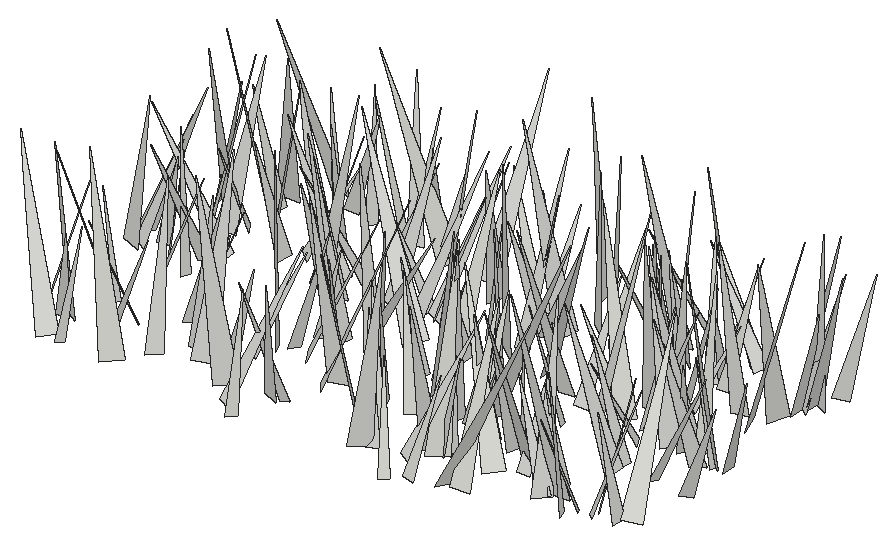
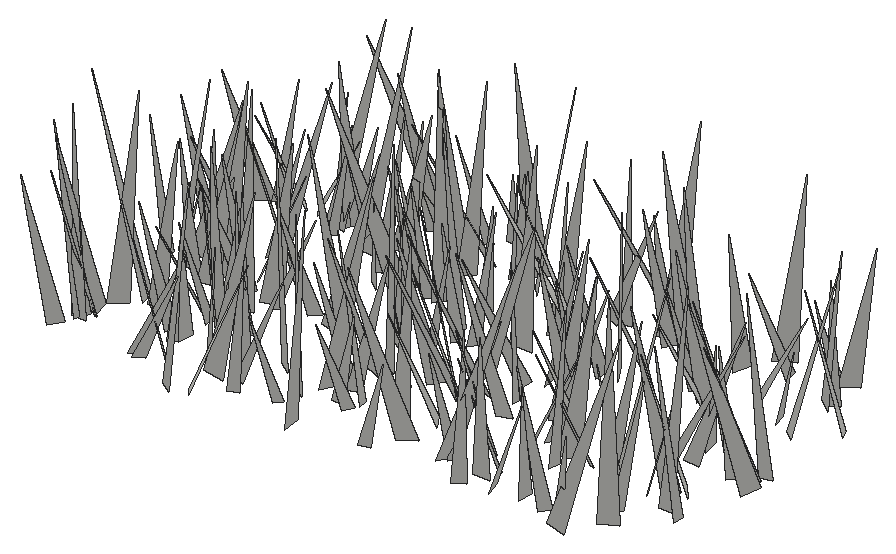
# SketchUp Ruby script. Lengths in inches.
U = 1.inch
M = Sketchup.active_model
def pt(a) = Geom::Point3d.new(a.map { |v| v * U })
def face(e, loops, mat)
  f = e.add_face(loops[0].map { |a| pt(a) })
  loops[1..].each { |l| e.add_face(l.map { |a| pt(a) }).erase! }
  f.material = f.back_material = mat if mat
  f
end
# faces: each face lists its corners as indices into pts; further lists are holes
def faces(e, pts, list, mat = nil) = list.each { |f| face(e, (f[0].is_a?(Array) ? f : [f]).map { |l| l.map { |i| pts[i] } }, mat) }
# xy, xz, yz: faces in a plane at the given z, y or x. An outline is a flat list of corners, or four numbers for a rectangle; further outlines are holes
def ring(l) = l.size == 4 ? [[l[0], l[1]], [l[2], l[1]], [l[2], l[3]], [l[0], l[3]]] : l.each_slice(2).to_a
def flat(e, list, mat, &to3) = list.each { |f| face(e, (f[0].is_a?(Array) ? f : [f]).map { |l| ring(l).map { |u, v| to3.(u, v) } }, mat) }
def xy(e, z, list, mat = nil) = flat(e, list, mat) { |x, y| [x, y, z] }
def xz(e, y, list, mat = nil) = flat(e, list, mat) { |x, z| [x, y, z] }
def yz(e, x, list, mat = nil) = flat(e, list, mat) { |y, z| [x, y, z] }
def lines(e, pts, list) = list.each { |a, b| e.add_line(pt(pts[a]), pt(pts[b])) }
# prism: a flat outline (further loops are holes) pulled along v
def prism(e, loops, v, mat = nil)
  f = face(e, loops, mat); d = Geom::Vector3d.new(v.map { |x| x * U })
  f.pushpull(f.normal.samedirection?(d) ? d.length : -d.length)
end
def box(e, o, s, mat = nil) = prism(e, [[o, [o[0] + s[0], o[1], o[2]], [o[0] + s[0], o[1] + s[1], o[2]], [o[0], o[1] + s[1], o[2]]]], [0, 0, s[2]], mat)
def at(x, y, z, deg = 0) = Geom::Transformation.translation(pt([x, y, z])) * Geom::Transformation.rotation(ORIGIN, Z_AXIS, deg.degrees)
def axes(o, x, y, z) = Geom::Transformation.new([*x, 0, *y, 0, *z, 0, *pt(o).to_a, 1])
def part(name) = M.definitions.add(name)
# library, detail: a bought-in or finely detailed component or shape, given as its bounding box
def library(name, o, s) = part(name).tap { |d| box(d.entities, o, s) }
def detail(e, o, s) = box(e.add_group.entities, o, s)
def put(e, d, t, mat = nil) = e.add_instance(d, t).tap { |i| i.material = mat if mat }
def group(e, t, mat = nil) = e.add_group.tap { |g| g.transformation = t; g.material = mat if mat }.entities
root = M.entities
c1 = part("fur_instance\#9")
p = [[0.8125,0,1.79],[0.67,-0.02,1.48],[0,-0.11,0],[0,0.11,0]]
faces(c1.entities,p,[[0,1,2,3]])
put(root,c1,axes([531.47,279.5,-21.66],[-0.67642,4.08917,0.12939],[3.98053,0.62749,0.97839],[-0.94522,-0.2838,4.0276]))
put(root,c1,axes([507.39,280.67,-21.66],[3.71191,-5.65782,4.04126],[-6.28277,-4.69165,-0.79764],[-2.97818,2.84578,6.7196]))
put(root,c1,axes([518.24,279.79,-21.66],[-3.95695,1.67084,0.9926],[1.45221,4.03835,-1.00857],[1.29152,0.5783,4.17516]))
put(root,c1,axes([532.73,280.46,-21.66],[0.16923,4.07191,1.2027],[4.12697,0.12503,-1.00402],[0.99752,-1.2081,3.94982]))
put(root,c1,axes([527.45,281.94,-21.66],[5.01911,-5.50348,2.14134],[-5.83765,-5.04831,0.7082],[-0.89193,2.07156,7.41473]))
put(root,c1,axes([518.71,283.35,-21.66],[-0.89521,-5.51634,1.09126],[-5.41102,1.14576,1.35291],[1.53027,0.82431,5.42227]))
put(root,c1,axes([501.875,280.69,-21.66],[-4.84886,5.21937,0.60309],[5.25064,4.78392,0.8135],[-0.19034,-0.99462,7.07753]))
put(root,c1,axes([503.04,280.5625,-21.66],[-3.70619,1.07071,1.22273],[0.63141,3.75399,-1.37341],[1.4976,1.06701,3.605]))
put(root,c1,axes([526.24,283.48,-21.66],[-5.36571,-5.00333,1.81378],[-4.95811,5.63559,0.87824],[1.93398,0.5664,7.28374]))
put(root,c1,axes([535.12,281.42,-21.66],[7.55011,-1.58138,0.22082],[-1.59514,-7.42262,1.38345],[0.0711,1.39915,7.58887]))
put(root,c1,axes([515.36,282.86,-21.66],[3.59874,-6.83955,3.08177],[-7.12327,-4.18751,-0.97538],[-2.35281,2.21652,7.66674]))
put(root,c1,axes([501.02,283.32,-21.66],[0.91273,-4.1627,0.50654],[-4.12867,-0.80133,0.85424],[0.734,0.66898,4.1751]))
put(root,c1,axes([516.92,280.75,-21.66],[2.4518,5.85296,0.01413],[5.81055,-2.43218,-0.76857],[0.70347,-0.30989,6.29903]))
put(root,c1,axes([531.23,284.64,-21.66],[5.68928,-3.36377,1.44998],[-3.11585,-5.85243,-1.35122],[-1.92583,-0.46842,6.46971]))
put(root,c1,axes([519.79,283.5625,-21.66],[-0.88602,-4.48963,1.06047],[-4.46813,0.56653,-1.33464],[-1.14769,1.26043,4.37728]))
put(root,c1,axes([505.84,282,-21.66],[4.17653,-0.25853,0.87813],[-0.4857,-4.1025,1.10224],[-0.77592,1.17643,4.03674]))
put(root,c1,axes([536.4,281.39,-21.66],[-1.26821,6.79621,1.34265],[6.86908,1.41065,-0.65215],[0.89826,-1.19212,6.8827]))
put(root,c1,axes([528.29,282.31,-21.66],[-1.05429,4.67357,0.99792],[4.75005,0.91265,0.74413],[-0.52453,-1.12891,4.73287]))
put(root,c1,axes([543.76,283.04,-21.66],[-4.56501,-1.69942,1.47091],[-1.97129,4.62695,-0.77219],[1.07964,1.26263,4.80947]))
put(root,c1,axes([514.65,283.77,-21.66],[3.82808,-2.96393,0.87418],[-3.08142,-3.76593,0.72521],[-0.23226,1.11183,4.78677]))
put(root,c1,axes([538.39,286.5,-21.66],[-2.04467,-7.63412,0.65301],[-7.56547,2.11851,1.07815],[1.21235,0.345,7.82931]))
put(root,c1,axes([542.29,284.84,-21.66],[-1.50167,-7.67594,2.08534],[-7.92089,1.24921,-1.10571],[-0.72669,2.24569,7.7429]))
put(root,c1,axes([501.56,283.66,-21.66],[-3.6941,-4.73944,2.34113],[-5.23892,3.66336,-0.85037],[0.70493,2.38895,5.94858]))
put(root,c1,axes([547.31,284.68,-21.66],[-4.17455,0.44699,1.70239],[0.80041,4.38471,0.81146],[1.56757,-1.04848,4.11925]))
put(root,c1,axes([544.33,284.09,-21.66],[-3.00148,-2.27694,0.1564],[-2.20162,2.82047,-1.1898],[-0.60148,1.03841,3.57459]))
put(root,c1,axes([532.32,284.51,-21.66],[2.08402,3.38406,1.47593],[3.68931,-1.84524,-0.97848],[0.13865,-1.76538,3.85196]))
put(root,c1,axes([541.26,284.22,-21.66],[-2.68831,3.38264,1.06218],[3.54497,2.54168,0.8778],[-0.06058,-1.37662,4.23069]))
put(root,c1,axes([530.9,282.5,-21.66],[2.76171,5.55128,0.00194],[5.48471,-2.72826,-0.95829],[0.85713,-0.42855,6.1258]))
put(root,c1,axes([528.06,283.32,-21.66],[-1.29816,5.29172,0.79515],[5.27739,1.13069,1.0911],[-0.88529,-1.01932,5.33826]))
put(root,c1,axes([508.99,283.17,-21.66],[-5.25856,3.05312,1.43062],[2.8843,5.44607,-1.02073],[1.74617,0.1987,5.99435]))
put(root,c1,axes([510.94,285.32,-21.66],[0.6303,-6.24139,2.24897],[-6.57772,-0.29373,1.02832],[0.86396,2.31708,6.18828]))
put(root,c1,axes([512.25,284.375,-21.66],[-3.47776,6.78239,3.15196],[7.08859,4.09761,-0.99596],[2.38486,-2.28893,7.55669]))
put(root,c1,axes([532.37,284.14,-21.66],[-5.26533,5.42334,2.66225],[5.51698,5.75546,-0.81326],[2.46233,-1.29842,7.51498]))
put(root,c1,axes([505.51,285.72,-21.66],[-2.7303,-2.91554,0.15676],[-2.8364,2.59761,-1.08937],[-0.69267,0.85529,3.84294]))
put(root,c1,axes([541.29,284.04,-21.66],[-5.91196,3.62871,1.99788],[3.48429,6.23911,-1.02156],[2.24027,-0.12769,6.86114]))
put(root,c1,axes([541.53,286.11,-21.66],[-3.71371,1.13934,1.58672],[1.47505,3.87017,0.67337],[1.28063,-1.15373,3.82574]))
put(root,c1,axes([498.09,285.93,-21.66],[4.56554,2.4835,0.72557],[2.58092,-4.47494,-0.92307],[-0.18188,-1.15993,5.11467]))
put(root,c1,axes([545.45,284.02,-21.66],[3.29969,3.36632,0.10349],[3.25213,-3.22241,1.12716],[-0.87548,0.71745,4.57707]))
put(root,c1,axes([532.77,285,-21.66],[1.28068,6.67783,2.12971],[6.86225,-1.63556,1.00185],[-1.42781,-1.87102,6.72532]))
put(root,c1,axes([536.59,284.75,-21.66],[-4.59485,5.55244,0.46156],[5.5505,4.50971,1.00485],[-0.48434,-0.99407,7.1367]))
put(root,c1,axes([535.84,287.96,-21.66],[4.30794,-3.29071,0.86204],[-3.07513,-4.36194,-1.28347],[-1.45447,-0.52435,5.26686]))
put(root,c1,axes([545.42,285,-21.66],[3.89268,2.82638,0.90518],[2.67493,-3.98806,0.94914],[-1.28551,0.26015,4.71599]))
put(root,c1,axes([500.9,288.33,-21.66],[-3.86726,-4.8383,0.71579],[-4.78645,3.93151,0.71436],[1.00566,0.10641,6.1526]))
put(root,c1,axes([534.05,287.73,-21.66],[4.56733,-2.95407,1.62637],[-2.80415,-4.84794,-0.93072],[-1.87305,0.05455,5.35918]))
put(root,c1,axes([525.3,287.41,-21.66],[-4.30625,-1.78107,2.16646],[-1.55574,4.81995,0.87021],[2.33354,-0.07334,4.57807]))
put(root,c1,axes([538.29,285.77,-21.66],[-1.13275,3.97734,1.11963],[3.98013,1.3621,-0.81189],[1.10966,-0.82546,4.05502]))
put(root,c1,axes([521.09,287.69,-21.66],[0.92373,-7.0899,2.33425],[-7.39568,-1.18748,-0.68009],[-1.00963,2.21177,7.11741]))
put(root,c1,axes([530.23,288.39,-21.66],[7.09602,-3.54407,1.49132],[-3.45875,-7.25092,-0.77408],[-1.67974,-0.04148,7.89397]))
put(root,c1,axes([520.56,288.54,-21.66],[-2.364,-4.99525,1.36106],[-4.8414,2.66304,1.36474],[1.83462,0.59091,5.35523]))
put(root,c1,axes([532.5,287.73,-21.66],[4.32257,0.5968,0.21737],[0.63053,-4.21214,-0.97382],[-0.07654,-0.99484,4.25352]))
put(root,c1,axes([508.21,288.06,-21.66],[4.08731,-3.32744,0.79787],[-3.41978,-4.01464,0.77613],[-0.11643,1.10699,5.21302]))
put(root,c1,axes([509.62,287.47,-21.66],[-0.91828,3.53646,1.4047],[3.57282,1.29857,-0.93362],[1.30946,-1.06309,3.53244]))
put(root,c1,axes([531.29,288.7,-21.66],[1.4619,-3.63585,0.57448],[-3.60479,-1.28901,1.01518],[0.74496,0.89757,3.78497]))
put(root,c1,axes([548.03,285.13,-21.66],[-3.4412,6.39637,0.09759],[6.32165,3.41718,-1.06042],[0.97968,0.41743,7.18546]))
put(root,c1,axes([502.64,287.15,-21.66],[-3.94683,-0.00707,0.27926],[-0.08275,3.80753,-1.07302],[0.26682,1.07619,3.79817]))
put(root,c1,axes([514.09,287.3,-21.66],[2.1149,3.97719,0.39309],[3.90996,-1.96694,-1.13523],[0.82754,-0.87089,4.35914]))
put(root,c1,axes([527.41,287.44,-21.66],[-1.32199,4.73147,0.88748],[4.77716,1.17578,0.84759],[-0.59431,-1.0737,4.83901]))
put(root,c1,axes([542.96,289.65,-21.66],[-6.41083,1.14128,1.69671],[1.48537,6.43646,1.28286],[1.40536,-1.59673,6.38401]))
put(root,c1,axes([520.5,286.49,-21.66],[5.97415,4.42308,0.10738],[4.35531,-5.91092,1.16532],[-0.77872,0.87356,7.3414]))
put(root,c1,axes([532.86,288.18,-21.66],[3.50267,-1.34823,2.1537],[-1.97697,-3.75014,0.86764],[-1.59615,1.68627,3.65152]))
put(root,c1,axes([532.64,288.06,-21.66],[-1.16488,5.07104,1.08343],[5.11451,1.30667,-0.61696],[0.85504,-0.90739,5.16641]))
put(root,c1,axes([548.65,290.19,-21.66],[3.25053,-3.28963,0.28157],[-3.26975,-3.15258,0.91484],[0.45796,0.84053,4.53329]))
put(root,c1,axes([517.09,289.33,-21.66],[5.75926,3.61485,0.22209],[3.58079,-5.62103,-1.36658],[0.54262,-1.27375,6.66098]))
put(root,c1,axes([514.87,288.86,-21.66],[-5.7993,-3.05465,2.69516],[-3.68736,5.92923,-1.21419],[1.7315,2.39584,6.44116]))
put(root,c1,axes([508.36,288.34,-21.66],[3.43862,2.40363,0.16823],[2.31203,-3.37399,0.94893],[-0.67841,0.6845,4.08669]))
put(root,c1,axes([515.74,289.65,-21.66],[4.66394,-1.20705,1.00362],[-1.36601,-4.67089,0.73033],[-0.77347,0.97077,4.76192]))
put(root,c1,axes([522.29,290.15,-21.66],[0.36283,-7.33481,3.26148],[-7.98321,-0.67122,-0.62142],[-0.83968,3.21222,7.31744]))
put(root,c1,axes([526.73,291.04,-21.66],[6.91292,1.02767,1.79019],[1.3308,-7.00178,-1.11957],[-1.57792,-1.40299,6.89863]))
put(root,c1,axes([542.87,290.79,-21.66],[-4.85785,0.78834,1.37895],[1.02249,4.94749,0.77364],[1.21552,-1.0112,4.86021]))
put(root,c1,axes([535.15,289.68,-21.66],[1.49909,3.09185,1.25062],[3.12666,-1.78006,0.6529],[-1.16087,-0.8017,3.3735]))
put(root,c1,axes([503.24,290.68,-21.66],[4.3525,2.53578,0.43229],[2.57081,-4.2585,-0.90411],[0.08934,-0.99816,4.9555]))
put(root,c1,axes([531.91,290.41,-21.66],[7.97011,-1.5942,0.50435],[-1.65185,-7.88792,1.1707],[-0.25934,1.24806,8.04323]))
put(root,c1,axes([524.85,291.9,-21.66],[4.20178,-1.75309,2.00996],[-1.5081,-4.65512,-0.90755],[-2.19975,-0.15714,4.46146]))
put(root,c1,axes([545.625,290.49,-21.66],[4.34496,-0.35551,0.43941],[-0.4633,-4.19131,1.19014],[-0.32376,1.22666,4.19388]))
put(root,c1,axes([526.01,292.125,-21.66],[2.52401,-3.24586,0.70539],[-3.32076,-2.44552,0.62916],[0.07602,0.94215,4.0633]))
put(root,c1,axes([516.17,291.78,-21.66],[2.59266,-2.6088,0.97622],[-2.78019,-2.50569,0.68761],[-0.17141,1.18171,3.61316]))
put(root,c1,axes([541.58,293.86,-21.66],[-3.32799,-2.15223,0.18164],[-2.02775,3.22824,1.09879],[0.74386,-0.82886,3.80792]))
put(root,c1,axes([546.8,293.73,-21.66],[0.96308,-5.75121,1.64983],[-5.7805,-1.32563,-1.24675],[-1.54408,1.37555,5.69645]))
put(root,c1,axes([536.19,292.65,-21.66],[-3.92472,-1.58946,0.29836],[-1.61245,3.78584,-1.04222],[-0.12416,1.07696,4.10409]))
put(root,c1,axes([517.86,292.41,-21.66],[-6.43885,-0.2283,0.73687],[-0.34147,6.39798,-1.00159],[0.69173,1.03328,6.36457]))
put(root,c1,axes([498.43,293.88,-21.66],[1.5633,5.69815,3.01797],[6.40687,-1.02237,-1.38843],[0.72737,-3.24142,5.74326]))
put(root,c1,axes([544.76,294.83,-21.66],[3.91329,-2.80057,0.16354],[-2.76188,-3.89534,-0.61821],[-0.49189,-0.40864,4.7723]))
put(root,c1,axes([503.64,295.26,-21.66],[0.77993,-5.26102,0.56712],[-5.12867,-0.89269,-1.22806],[-1.30258,0.36472,5.1748]))
put(root,c1,axes([548.64,294.72,-21.66],[4.67229,-0.63233,0.28263],[-0.57173,-4.60903,-0.86025],[-0.39095,-0.81674,4.63574]))
put(root,c1,axes([503.98,292.79,-21.66],[-5.02502,0.15502,0.9974],[-0.08895,4.97687,-1.22169],[1.00545,1.21508,4.87671]))
put(root,c1,axes([500.14,295.25,-21.66],[2.04033,-4.0488,0.48109],[-4.03745,-1.93127,0.8697],[0.56854,0.81522,4.44965]))
put(root,c1,axes([525.71,295.68,-21.66],[-3.46561,0.71078,2.1355],[1.4755,3.67824,1.17025],[1.69955,-1.74395,3.33859]))
put(root,c1,axes([543.7,294.89,-21.66],[-5.4764,4.5647,2.90915],[5.14181,5.68019,0.76664],[1.69155,-2.48788,7.08799]))
put(root,c1,axes([518.8,294.01,-21.66],[4.72114,-1.50275,0.05764],[-1.46013,-4.53503,1.361],[0.36002,1.31378,4.76394]))
put(root,c1,axes([547.63,294.51,-21.66],[-4.59653,-5.39297,2.39685],[-5.86856,4.49796,-1.13384],[0.62378,2.57709,6.99476]))
put(root,c1,axes([533.8,296.05,-21.66],[-0.89834,-6.55906,1.37521],[-6.65422,0.70817,-0.96916],[-0.7961,1.48213,6.54897]))
put(root,c1,axes([547.69,294.23,-21.66],[-3.7674,-0.4134,0.34529],[-0.49063,3.64055,-0.99453],[0.22227,1.02903,3.6572]))
put(root,c1,axes([501.4,294.21,-21.66],[-2.88957,-1.62735,2.00469],[-2.2228,3.09866,-0.68855],[1.31385,1.66334,3.24403]))
put(root,c1,axes([543.88,296.44,-21.66],[2.81422,-5.9892,1.8303],[-5.99838,-3.15452,-1.09945],[-1.79999,1.14839,6.52546]))
put(root,c1,axes([517.93,296.11,-21.66],[4.34491,0.59069,1.09524],[0.90101,-4.23706,-1.28924],[-0.85828,-1.45776,4.19106]))
put(root,c1,axes([512.7,296.94,-21.66],[2.86729,-4.50295,0.62999],[-4.43501,-2.93396,-0.78577],[-1.00209,0.10064,5.2802]))
put(root,c1,axes([498.9,294.22,-21.66],[2.45412,4.72767,0.6627],[4.74881,-2.3413,-0.8831],[0.48874,-0.99004,5.25297]))
put(root,c1,axes([513.9375,296.49,-21.66],[1.75802,-6.33898,1.96931],[-6.51413,-2.03906,-0.74828],[-1.27556,1.67662,6.53555]))
put(root,c1,axes([529.01,294.93,-21.66],[1.89742,4.59885,2.05217],[4.78177,-2.33318,0.8074],[-1.57969,-1.53878,4.90894]))
put(root,c1,axes([504.62,296.39,-21.66],[-6.1435,0.43905,0.01492],[0.43419,6.03663,1.1429],[-0.06685,-1.14104,6.05221]))
put(root,c1,axes([541.01,295.6,-21.66],[4.40781,-2.35415,1.32075],[-2.57038,-4.43283,0.67704],[-0.82436,1.23418,4.95101]))
put(root,c1,axes([538.34,296.3,-21.66],[-3.99734,1.08155,0.32432],[1.12476,3.91891,0.79421],[0.09918,-0.85212,4.0642]))
put(root,c1,axes([498.08,295.875,-21.66],[6.2285,-2.9564,0.62521],[-3.02175,-6.08711,1.31964],[0.01382,1.46019,6.76705]))
put(root,c1,axes([538.09,293.75,-21.66],[3.95249,6.61953,0.92655],[6.54498,-4.05132,1.02412],[-1.35642,-0.25967,7.64143]))
put(root,c1,axes([539.79,297.64,-21.66],[-0.40221,-7.56998,1.93164],[-7.73436,0.65878,0.97125],[1.10251,1.85984,7.51818]))
put(root,c1,axes([521.65,295.14,-21.66],[-7.18183,4.15456,0.03319],[4.14203,7.15453,0.70461],[-0.3242,-0.62648,8.26695]))
put(root,c1,axes([535.7,295.24,-21.66],[-1.59343,4.55905,1.08338],[4.45907,1.82697,-1.12985],[1.44061,-0.61229,4.69546]))
put(root,c1,axes([530.95,297.67,-21.66],[7.51831,-0.309,0.51299],[-0.23256,-7.46002,-1.08516],[-0.55186,-1.06592,7.446]))
put(root,c1,axes([527.25,297.87,-21.66],[-3.84702,-6.56229,2.86732],[-6.71624,4.43571,1.14075],[2.48541,1.82909,7.52076]))
put(root,c1,axes([538.89,295.8125,-21.66],[2.27452,-5.56414,4.58515],[-6.58849,-3.55674,-1.04785],[-2.92831,3.68058,5.91904]))
put(root,c1,axes([541.07,295.83,-21.66],[4.54007,-1.04122,1.07478],[-1.33062,-4.37982,1.37772],[-0.68465,1.60765,4.44952]))
put(root,c1,axes([545.71,295.54,-21.66],[0.35449,6.1752,1.09899],[6.2119,-0.49795,0.79425],[-0.86782,-1.04187,6.13416]))
put(root,c1,axes([507.69,298.61,-21.66],[-4.50462,1.14541,2.32905],[1.86637,4.67145,1.31236],[1.80364,-1.97324,4.45884]))
put(root,c1,axes([512.69,298.7,-21.66],[-6.22259,1.31552,1.1088],[1.51746,6.15727,1.21077],[0.81078,-1.42761,6.24382]))
put(root,c1,axes([541.85,296.71,-21.66],[-4.80614,1.67739,0.07303],[1.63862,4.73444,-0.90443],[0.36591,0.83033,5.00945]))
put(root,c1,axes([513.59,299.72,-21.66],[-4.70083,-1.74871,0.0814],[-1.70109,4.61801,0.97093],[0.41342,-0.88228,4.92068]))
put(root,c1,axes([512.04,297.14,-21.66],[6.62959,-1.41825,2.66639],[-1.99694,-6.88369,1.30369],[-2.26567,1.91728,6.65307]))
put(root,c1,axes([519.67,299.29,-21.66],[-3.46593,0.7925,0.89611],[1.04093,3.35143,1.06213],[0.58952,-1.25841,3.39303]))
put(root,c1,axes([520.2,296.52,-21.66],[2.81698,6.47491,0.35167],[6.46114,-2.77024,-0.75032],[0.54938,-0.62035,7.02117]))
put(root,c1,axes([523.62,297.37,-21.66],[-3.09006,5.24053,1.65653],[5.13422,3.43055,-1.27548],[1.9614,-0.72379,5.94851]))
put(root,c1,axes([506.57,299.3,-21.66],[-6.42891,-4.93695,1.78859],[-5.18873,6.40682,-0.96596],[0.80598,1.86616,8.04806]))
put(root,c1,axes([503.27,300.42,-21.66],[-3.15969,-2.10838,0.70871],[-1.88389,3.19122,1.09464],[1.18257,-0.54957,3.6374]))
put(root,c1,axes([540.09,299.91,-21.66],[0.10364,-5.95888,1.80759],[-6.13378,0.21397,1.05707],[1.07352,1.79787,5.86529]))
put(root,c1,axes([521.94,297.48,-21.66],[5.36611,5.59511,2.05394],[5.5109,-5.71038,1.15783],[-2.27022,-0.63666,7.66549]))
put(root,c1,axes([520.3,298.75,-21.66],[4.29759,3.17988,0.45483],[3.21134,-4.23507,-0.73441],[0.07624,-0.86047,5.29543]))
put(root,c1,axes([517.2,298.18,-21.66],[0.34617,6.42334,1.62872],[6.51894,-0.03728,-1.2385],[1.18972,-1.66468,6.31231]))
put(root,c1,axes([510.375,299.8,-21.66],[-3.35147,5.54659,2.9979],[6.27053,3.28643,0.92965],[0.65767,-3.06906,6.41348]))
put(root,c1,axes([500.9,301.36,-21.66],[-1.7083,-7.51191,1.45388],[-7.48357,1.95063,1.28533],[1.59333,1.10775,7.59572]))
put(root,c1,axes([510.85,297.48,-21.66],[4.46685,2.95329,0.59597],[2.75098,-4.43263,1.34675],[-1.2285,0.81223,5.18275]))
put(root,c1,axes([539.26,298.79,-21.66],[-4.67336,-1.61213,2.14084],[-2.03116,4.93814,-0.71533],[1.7483,1.42769,4.89159]))
put(root,c1,axes([502.27,299.17,-21.66],[-0.87926,6.56228,2.62812],[6.83144,1.46959,-1.38397],[1.81713,-2.34956,6.47466]))
put(root,c1,axes([525.14,298.42,-21.66],[2.28996,3.33239,0.84649],[3.03653,-2.43723,1.38011],[-1.61271,0.14282,3.80053]))
put(root,c1,axes([546.94,302.08,-21.66],[6.05759,-4.04132,1.47541],[-3.82561,-6.22554,-1.34569],[-1.96821,-0.33746,7.15653]))
put(root,c1,axes([545.92,300.32,-21.66],[7.78659,2.72532,1.24866],[2.87625,-7.77148,-0.97412],[-0.84485,-1.33952,8.19204]))
put(root,c1,axes([508.52,299.76,-21.66],[2.58495,3.56171,0.23056],[3.43761,-2.40789,-1.34382],[0.96012,-0.96809,4.1907]))
put(root,c1,axes([527.24,301.65,-21.66],[2.70621,-3.86796,1.26709],[-3.69816,-2.97221,-1.17466],[-1.70008,0.30833,4.57219]))
put(root,c1,axes([510.52,301.28,-21.66],[5.22033,-0.21574,2.13038],[0.1303,-5.5713,-0.88347],[-2.13731,-0.86658,5.14955]))
put(root,c1,axes([501.4,298.52,-21.66],[4.49985,4.45709,1.03745],[4.28289,-4.6143,1.2473],[-1.61209,0.1822,6.20956]))
put(root,c1,axes([541.65,299.67,-21.66],[1.90499,3.12749,0.05078],[3.06447,-1.8542,-0.76405],[0.62675,-0.43991,3.5814]))
put(root,c1,axes([520.53,298.56,-21.66],[1.99959,6.47326,0.24716],[6.43471,-1.95494,-0.85747],[0.74746,-0.48749,6.72058]))
put(root,c1,axes([544.51,301.06,-21.66],[-0.07394,-6.12578,2.47714],[-6.56947,-0.19789,-0.68546],[-0.70961,2.47033,6.08776]))
put(root,c1,axes([499.51,301.83,-21.66],[5.83398,1.13984,1.03884],[1.35175,-5.73614,-1.2974],[-0.74243,-1.48703,5.80098]))
put(root,c1,axes([527.8,301.2,-21.66],[3.87779,-2.1954,0.31482],[-2.2129,-3.78759,0.8446],[0.14815,0.88911,4.37535]))
put(root,c1,axes([540.71,300.22,-21.66],[4.041,0.55824,1.1889],[0.26805,-4.11576,1.02147],[-1.28579,0.89645,3.94942]))
put(root,c1,axes([532.84,302.01,-21.66],[-4.52397,-6.09316,3.51067],[-6.34353,5.33763,1.08955],[3.03497,2.07386,7.51038]))
put(root,c1,axes([522.19,303.03,-21.66],[5.38586,-3.00561,1.16634],[-2.8404,-5.49795,-1.05176],[-1.52519,-0.37466,6.07741]))
put(root,c1,axes([528.85,302.18,-21.66],[-7.80525,1.8691,2.4402],[2.24771,8.01322,1.05174],[2.09664,-1.63243,7.95672]))
put(root,c1,axes([537.33,300.34,-21.66],[-3.18847,2.06393,0.29466],[1.98964,3.17316,-0.69666],[0.62286,0.42918,3.73374]))
put(root,c1,axes([527.66,298.9,-21.66],[1.84381,6.83005,0.32521],[6.75707,-1.87158,0.99709],[-1.04756,-0.05069,7.00393]))
put(root,c1,axes([525.7,302.625,-21.66],[5.69454,1.71793,1.14191],[1.95584,-5.5622,-1.38552],[-0.6557,-1.67144,5.78441]))
put(root,c1,axes([535.42,303,-21.66],[5.69502,0.05498,1.49404],[0.36012,-5.7612,-1.16071],[-1.45103,-1.21405,5.57575]))
put(root,c1,axes([504.93,301.13,-21.66],[4.32331,2.64676,1.47041],[2.57631,-4.56233,0.63737],[-1.59061,-0.19566,5.02892]))
put(root,c1,axes([540.91,303.9,-21.66],[3.64038,-1.44849,0.64201],[-1.22649,-3.59476,-1.15586],[-1.003,-0.8615,3.74359]))
put(root,c1,axes([503.36,303.55,-21.66],[-4.62696,1.13691,1.70574],[1.48296,4.76376,0.84751],[1.41525,-1.27471,4.68861]))
put(root,c1,axes([502.73,305.24,-21.66],[1.80193,-7.44469,0.50754],[-7.36471,-1.69029,1.35351],[1.20089,0.80465,7.53912]))
put(root,c1,axes([520.26,301.47,-21.66],[4.1336,3.03674,0.5342],[2.87698,-4.11997,1.15876],[-1.10914,0.6308,4.99657]))
put(root,c1,axes([541.75,302.85,-21.66],[-1.54169,4.36128,2.00643],[4.43238,2.10262,-1.16464],[1.84406,-1.40768,4.47674]))
put(root,c1,axes([537.59,304.19,-21.66],[-1.86728,-3.21645,1.13397],[-3.16749,2.11482,0.78275],[1.26429,0.54787,3.63587]))
put(root,c1,axes([530.01,304.06,-21.66],[-3.26006,-5.04679,2.60885],[-5.29814,3.78652,0.70434],[2.05082,1.75965,5.96674]))
put(root,c1,axes([547.6875,304.96,-21.66],[6.64533,-1.36705,0.39109],[-1.31179,-6.61549,-0.83466],[-0.54862,-0.74069,6.73295]))
put(root,c1,axes([534.12,305.31,-21.66],[-0.56318,-3.80765,0.20803],[-3.75255,0.51599,-0.71463],[-0.67806,0.30692,3.78215]))
put(root,c1,axes([515.02,302.22,-21.66],[1.99951,5.4557,0.6063],[5.41529,-2.06607,0.73224],[-0.89823,-0.31139,5.76424]))
put(root,c1,axes([516.68,304.98,-21.66],[-8.04315,1.60644,1.39343],[1.83623,7.99603,1.38066],[1.07265,-1.64234,8.08496]))
put(root,c1,axes([547.78,305.25,-21.66],[-1.4348,-7.0433,2.45033],[-7.23254,1.92235,1.29061],[1.81726,2.08982,7.07114]))
put(root,c1,axes([512.89,304.08,-21.66],[2.48404,3.35431,0.63876],[3.34518,-2.23213,-1.28736],[0.685,-1.26336,3.97047]))
put(root,c1,axes([527.1,303.48,-21.66],[-1.4583,4.1794,0.64732],[4.14586,1.27741,1.09233],[-0.83566,-0.95598,4.28962]))
put(root,c1,axes([540.46,303.02,-21.66],[-4.55116,2.07867,0.64916],[1.93391,4.54938,-1.00919],[1.00113,0.66152,4.90056]))
put(root,c1,axes([547.33,303.54,-21.66],[6.67173,1.075,1.66778],[0.88806,-6.84957,0.86244],[-1.77439,0.61387,6.70252]))
put(root,c1,axes([536.15,304.79,-21.66],[-4.08433,-4.26667,3.28401],[-4.58243,4.91876,0.69141],[2.82675,1.80893,5.86585]))
put(root,c1,axes([536.89,304.07,-21.66],[0.66208,3.60921,1.19442],[3.54519,-1.02396,1.12897],[-1.37285,-0.90361,3.49144]))
put(root,c1,axes([533.46,306.69,-21.66],[0.2783,-5.0487,0.14304],[-4.93686,-0.24166,1.07529],[1.0664,0.19877,4.94071]))
put(root,c1,axes([547.35,304.2,-21.66],[2.91311,4.64162,1.0633],[4.76072,-2.81168,-0.76908],[0.10392,-1.30816,5.4258]))
put(root,c1,axes([516.2,304.74,-21.66],[-1.839,3.01934,1.93742],[3.07994,2.44517,-0.88715],[1.83955,-1.07548,3.42218]))
put(root,c1,axes([526.01,303.82,-21.66],[-2.24412,3.20659,0.81725],[3.00578,2.38826,-1.11699],[1.38398,0.01256,3.75108]))
put(root,c1,axes([535.91,305.8125,-21.66],[-0.62718,-6.98929,2.39617],[-7.29856,0.2117,-1.29283],[-1.15016,2.46782,6.89725]))
put(root,c1,axes([513.98,307.09,-21.66],[1.58205,-4.94043,0.08132],[-4.90313,-1.55912,0.66773],[0.6114,0.28046,5.1444]))
put(root,c1,axes([507.17,306.39,-21.66],[2.31038,-4.41979,0.71264],[-4.3801,-2.06578,1.38834],[0.92579,1.25629,4.79008]))
put(root,c1,axes([505.16,307.86,-21.66],[-0.75565,-7.24529,1.23648],[-7.25287,0.53359,-1.30585],[-1.19119,1.34729,7.16659]))
put(root,c1,axes([541.84,306.67,-21.66],[-4.37284,2.10544,0.41102],[2.13916,4.20984,1.19366],[-0.16073,-1.25217,4.70423]))
put(root,c1,axes([513.35,305.52,-21.66],[-0.65155,5.99766,1.58433],[6.18323,0.49957,0.65163],[-0.49968,-1.63861,5.99765]))
put(root,c1,axes([509.35,305.82,-21.66],[-4.59387,1.36569,1.34916],[1.20913,4.77619,-0.71765],[1.49109,0.33451,4.73854]))
put(root,c1,axes([535.74,308.62,-21.66],[-3.80651,-3.12707,0.03174],[-3.06593,3.74155,0.93273],[0.61617,-0.70095,4.83716]))
put(root,c1,axes([538.64,307.12,-21.66],[3.81482,2.67004,0.71919],[2.75746,-3.58156,-1.32965],[0.20681,-1.49748,4.4625]))
put(root,c1,axes([530.23,306,-21.66],[-1.29453,3.3269,0.92168],[3.25121,1.50588,-0.8692],[1.16077,-0.50757,3.46245]))
put(root,c1,axes([548.49,306.79,-21.66],[3.34726,-4.07819,1.53745],[-4.35777,-3.09938,1.26621],[0.07255,1.99042,5.12177]))
put(root,c1,axes([520.33,304.61,-21.66],[-1.86477,7.56726,1.18834],[7.49142,2.05683,-1.34204],[1.5982,-0.81177,7.67722]))
put(root,c1,axes([511.8,306.2,-21.66],[-4.83845,-0.36416,0.05457],[-0.36621,4.6838,-1.21411],[-0.03844,1.21473,4.69778]))
put(root,c1,axes([527.66,307.8,-21.66],[-7.27615,-1.41209,3.18772],[-1.2687,7.94356,0.62294],[3.24745,-0.06052,7.38568]))
put(root,c1,axes([505.96,306.49,-21.66],[0.1057,3.9764,0.92499],[3.9126,-0.36287,1.11284],[-1.16573,-0.85739,3.81897]))
put(root,c1,axes([541.29,306.99,-21.66],[-3.62089,2.64212,0.01483],[2.58278,3.53416,0.96476],[-0.55698,-0.78788,4.37731]))
put(root,c1,axes([522.07,307.05,-21.66],[-2.23276,3.13779,0.67741],[3.20125,2.1153,0.75324],[-0.23799,-0.9847,3.77672]))
put(root,c1,axes([537.34,309.04,-21.66],[-4.05006,-5.82532,2.03849],[-5.82326,4.4146,1.04584],[2.04438,1.03428,7.01738]))
